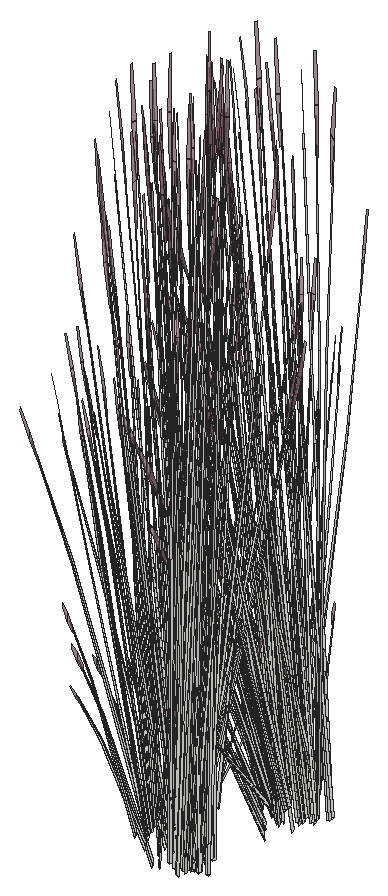
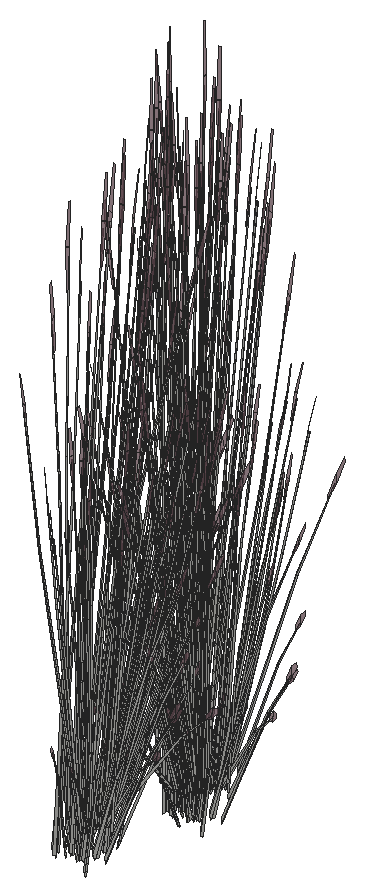
# SketchUp Ruby script. Lengths in inches.
U = 1.inch
M = Sketchup.active_model
def pt(a) = Geom::Point3d.new(a.map { |v| v * U })
def face(e, loops, mat)
  f = e.add_face(loops[0].map { |a| pt(a) })
  loops[1..].each { |l| e.add_face(l.map { |a| pt(a) }).erase! }
  f.material = f.back_material = mat if mat
  f
end
# faces: each face lists its corners as indices into pts; further lists are holes
def faces(e, pts, list, mat = nil) = list.each { |f| face(e, (f[0].is_a?(Array) ? f : [f]).map { |l| l.map { |i| pts[i] } }, mat) }
# xy, xz, yz: faces in a plane at the given z, y or x. An outline is a flat list of corners, or four numbers for a rectangle; further outlines are holes
def ring(l) = l.size == 4 ? [[l[0], l[1]], [l[2], l[1]], [l[2], l[3]], [l[0], l[3]]] : l.each_slice(2).to_a
def flat(e, list, mat, &to3) = list.each { |f| face(e, (f[0].is_a?(Array) ? f : [f]).map { |l| ring(l).map { |u, v| to3.(u, v) } }, mat) }
def xy(e, z, list, mat = nil) = flat(e, list, mat) { |x, y| [x, y, z] }
def xz(e, y, list, mat = nil) = flat(e, list, mat) { |x, z| [x, y, z] }
def yz(e, x, list, mat = nil) = flat(e, list, mat) { |y, z| [x, y, z] }
def lines(e, pts, list) = list.each { |a, b| e.add_line(pt(pts[a]), pt(pts[b])) }
# prism: a flat outline (further loops are holes) pulled along v
def prism(e, loops, v, mat = nil)
  f = face(e, loops, mat); d = Geom::Vector3d.new(v.map { |x| x * U })
  f.pushpull(f.normal.samedirection?(d) ? d.length : -d.length)
end
def box(e, o, s, mat = nil) = prism(e, [[o, [o[0] + s[0], o[1], o[2]], [o[0] + s[0], o[1] + s[1], o[2]], [o[0], o[1] + s[1], o[2]]]], [0, 0, s[2]], mat)
def at(x, y, z, deg = 0) = Geom::Transformation.translation(pt([x, y, z])) * Geom::Transformation.rotation(ORIGIN, Z_AXIS, deg.degrees)
def axes(o, x, y, z) = Geom::Transformation.new([*x, 0, *y, 0, *z, 0, *pt(o).to_a, 1])
def part(name) = M.definitions.add(name)
# library, detail: a bought-in or finely detailed component or shape, given as its bounding box
def library(name, o, s) = part(name).tap { |d| box(d.entities, o, s) }
def detail(e, o, s) = box(e.add_group.entities, o, s)
def put(e, d, t, mat = nil) = e.add_instance(d, t).tap { |i| i.material = mat if mat }
def group(e, t, mat = nil) = e.add_group.tap { |g| g.transformation = t; g.material = mat if mat }.entities
root = M.entities
M.materials.add("LightPink_Translucent").color = [144, 107, 117]
M.materials["LightPink_Translucent"].alpha = 0.75
c1 = part("blade")
p = [[2.15,0.21,22],[0,0.17,0],[0.09,0.45,0],[2.18,0.31,22],[2.29,0.31,22],[0.38,0.45,0],
  [2.48,0.24,33],[2.49,0.24,33],[2.48,0.22,33]]
faces(c1.entities,p,[[0,1,2,3],[4,5,2,3],[6,3,4,7],[8,0,3,6]])
c2 = part("seeds")
p = [[0.3,-0.1,1.38],[-0.01,-0.03,1.59],[-0.01,-0.03,0.03],[0.14,-0.07,-0.07],[0.29,-0.03,3],[0.15,0.01,3.11]]
faces(c2.entities,p,[[0,1,2,3],[1,0,4,5]],"LightPink_Translucent")
c3 = part("blade with seeds")
put(c3.entities,c1,at(0,0,0))
put(c3.entities,c2,axes([2.4,0.25,30.99],[1.5799,-0.05474,1.17369],[-0.12525,1.92788,0.29478],[-0.07173,-0.02425,1.56792]))
put(root,c3,axes([316.24,325.63,275.875],[0.20841,-0.0122,1.71376],[-0.13825,0.52864,0.13857],[-0.297,-0.0327,0.73262]))
put(root,c3,axes([316.33,326.56,275.875],[0.17434,-0.11391,1.71376],[0.14677,0.52637,0.13857],[-0.27369,0.11897,0.73262]))
put(root,c3,axes([315.78,327.46,274.59],[0.17462,0.04421,1.43002],[0.11254,0.45156,-0.30754],[-0.23719,0.08453,0.61141]))
put(root,c3,axes([317.33,326.01,275.34],[0.14282,-0.0779,1.77064],[0.04925,0.54394,0.13857],[-0.30935,0.07218,0.63284]))
put(root,c3,axes([315.79,326.375,276.72],[-0.08205,0.06992,1.74944],[0.00698,0.51086,-0.27667],[-0.18807,0.06644,0.14031]))
put(root,c3,axes([316.06,326.08,276.53],[-0.41757,-0.15024,-0.35414],[0.12179,-0.4383,0.4572],[-0.16812,0.04019,0.87481]))
put(root,c3,axes([314.88,326.89,276.71],[0.06412,0.01444,1.77383],[0.19837,0.47583,-0.16761],[-0.13126,0.12489,0.31391]))
put(root,c3,axes([316.34,326.31,276.68],[-0.13612,0.48987,-0.51099],[-0.46669,-0.16791,-0.3958],[-0.1879,0.04492,0.97773]))
put(root,c3,axes([316.7,325.25,276.68],[-0.36484,0.35674,-0.51099],[-0.31952,-0.37685,-0.3958],[-0.18537,-0.05428,0.97773]))
put(root,c3,axes([316.11,326.28,273.49],[0.01274,0.08487,1.76342],[-0.25688,0.44323,-0.26939],[-0.18246,-0.02234,0.30037]))
put(root,c3,axes([316.18,324.25,276.71],[0.03725,0.05374,1.77383],[-0.17957,0.48312,-0.16761],[-0.18186,0.0035,0.31391]))
put(root,c3,axes([315.42,328.4,274.77],[0.2094,-0.24408,1.1486],[0.08263,0.38639,0.84392],[-0.15132,0.06919,0.25299]))
put(root,c3,axes([316.15,326.03,276.73],[0.14195,-0.49104,0.48003],[0.46669,0.16791,0.3958],[-0.18353,0.02951,0.9933]))
put(root,c3,axes([316.32,325.89,277.03],[0.25281,0.48765,-0.1216],[-0.44869,0.23964,-0.67495],[-0.18908,0.06434,1.02557]))
put(root,c3,axes([316.89,324.875,277.03],[-0.0269,0.54769,-0.1216],[-0.50939,-0.01497,-0.67495],[-0.19618,-0.03804,1.02557]))
put(root,c3,axes([316.12,325.9,276.73],[-0.18454,-0.3672,0.0643],[0.33652,-0.17973,0.50621],[-0.14834,0.03546,0.77189]))
put(root,c3,axes([316.96,326.91,275.875],[0.1255,-0.16547,1.71376],[0.31687,0.44665,0.13857],[-0.21734,0.2034,0.73262]))
put(root,c3,axes([316.21,327.35,276.53],[-0.43736,0.07697,-0.35414],[-0.11549,-0.43998,0.4572],[-0.12533,0.11818,0.87481]))
put(root,c3,axes([315.97,328.65,273.49],[0.0674,0.0538,1.76342],[0.11428,0.49852,-0.26939],[-0.14937,0.10631,0.30037]))
put(root,c3,axes([315.875,325.72,274.77],[0.32078,-0.03854,1.1486],[-0.20348,0.33954,0.84392],[-0.15852,-0.05093,0.25299]))
put(root,c3,axes([316.27,327.25,276.73],[-0.12461,-0.49565,0.48003],[0.48882,-0.08602,0.3958],[-0.14406,0.11657,0.9933]))
put(root,c3,axes([316.17,327.16,276.73],[-0.34493,-0.22649,0.0643],[0.20082,-0.32253,0.50621],[-0.11059,0.10427,0.77189]))
put(root,c3,axes([316.87,327.32,275.875],[0.09355,-0.18511,1.71376],[0.39247,0.38307,0.13857],[-0.17705,0.23875,0.73262]))
put(root,c3,axes([316.5,326.03,277.05],[0.41757,0.15024,0.35414],[-0.12179,0.4383,-0.4572],[-0.16812,0.04019,0.87481]))
put(root,c3,axes([319.15,335.58,275.875],[0.20841,-0.0122,1.71376],[-0.13825,0.52864,0.13857],[-0.297,-0.0327,0.73262]))
put(root,c3,axes([316.57,327.4,276.68],[0.12908,0.49174,-0.51099],[-0.48882,0.08602,-0.3958],[-0.14008,0.13208,0.97773]))
put(root,c3,axes([315.81,328.28,276.72],[-0.01249,0.10657,1.74944],[0.35444,0.37075,-0.27667],[-0.09279,0.17532,0.14031]))
put(root,c3,axes([317.79,327.05,274.06],[-0.52267,-0.08829,-0.62353],[0.11029,-0.54463,-0.16365],[-0.15598,-0.06599,1.37633]))
put(root,c3,axes([316.97,325.09,277.05],[0.28589,0.33718,0.35414],[-0.32644,0.31919,-0.4572],[-0.16586,-0.04856,0.87481]))
put(root,c3,axes([317.1,328.08,274.02],[-0.47024,-0.26927,-0.49651],[0.28107,-0.48284,0],[-0.1071,-0.06133,1.57504]))
put(root,c3,axes([319.24,336.51,275.875],[0.17434,-0.11391,1.71376],[0.14677,0.52637,0.13857],[-0.27369,0.11897,0.73262]))
put(root,c3,axes([316.34,327.05,277.03],[0.46478,0.29695,-0.1216],[-0.26776,0.43004,-0.67495],[-0.13131,0.14949,1.02557]))
put(root,c3,axes([317.39,328.4,274.375],[-0.31414,0.53965,0],[-0.52557,-0.30095,-0.51607],[-0.1197,-0.06854,1.63711]))
put(root,c3,axes([318.7,337.4,274.59],[0.17462,0.04421,1.43002],[0.11254,0.45156,-0.30754],[-0.23719,0.08453,0.61141]))
put(root,c3,axes([320.24,335.96,275.34],[0.14282,-0.0779,1.77064],[0.04925,0.54394,0.13857],[-0.30935,0.07218,0.63284]))
put(root,c3,axes([315.57,328.34,277.65],[0.44338,0.14375,-0.06488],[-0.13639,0.44245,-0.29416],[-0.07252,0.06718,0.97024]))
put(root,c3,axes([316.57,327.09,277.05],[0.43736,-0.07697,0.35414],[0.11549,0.43998,-0.4572],[-0.12533,0.11818,0.87481]))
put(root,c3,axes([316.82,329.18,274.59],[0.15856,-0.08496,1.43002],[0.39147,0.25616,-0.30754],[-0.11652,0.22165,0.61141]))
put(root,c3,axes([318.7,336.32,276.72],[-0.08205,0.06992,1.74944],[0.00698,0.51086,-0.27667],[-0.18807,0.06644,0.14031]))
put(root,c3,axes([319.77,335.08,276.98],[-0.50227,-0.01297,-0.71045],[0.03373,-0.54602,0.08574],[-0.21278,-0.05762,1.00501]))
put(root,c3,axes([319.37,335.22,274.59],[0.0981,0.14994,1.43002],[-0.22605,0.40756,-0.30754],[-0.23211,-0.09741,0.61141]))
put(root,c3,axes([318.38,327.125,274.67],[-0.5073,0.35754,-0.29095],[-0.33735,-0.5052,-0.50002],[-0.12516,-0.05131,1.59708]))
put(root,c3,axes([318.97,336.03,276.53],[-0.41757,-0.15024,-0.35414],[0.12179,-0.4383,0.4572],[-0.16812,0.04019,0.87481]))
put(root,c3,axes([316.98,328.25,276.73],[-0.35779,-0.36745,0.48003],[0.37996,-0.3169,0.3958],[-0.066,0.17239,0.9933]))
put(root,c3,axes([319.55,334.73,275.875],[0.18664,0.09279,1.71376],[-0.38624,0.38925,0.13857],[-0.24072,-0.1756,0.73262]))
put(root,c3,axes([317.23,327.875,274.03],[-0.11803,-0.46926,-0.30978],[0.46876,-0.13325,0.30978],[-0.0945,-0.05411,1.38974]))
put(root,c3,axes([316.85,328.22,276.73],[-0.4129,-0.02509,0.0643],[0.01132,-0.37891,0.50621],[-0.04321,0.14514,0.77189]))
put(root,c3,axes([316.98,328.37,276.53],[-0.33997,0.28354,-0.35414],[-0.32182,-0.32376,0.4572],[-0.04897,0.1645,0.87481]))
put(root,c3,axes([317.79,336.84,276.71],[0.06412,0.01444,1.77383],[0.19837,0.47583,-0.16761],[-0.13126,0.12489,0.31391]))
put(root,c3,axes([319.25,336.25,276.68],[-0.13612,0.48987,-0.51099],[-0.46669,-0.16791,-0.3958],[-0.1879,0.04492,0.97773]))
put(root,c3,axes([319.61,335.19,276.68],[-0.36484,0.35674,-0.51099],[-0.31952,-0.37685,-0.3958],[-0.18537,-0.05428,0.97773]))
put(root,c3,axes([319.02,336.22,273.49],[0.01274,0.08487,1.76342],[-0.25688,0.44323,-0.26939],[-0.18246,-0.02234,0.30037]))
put(root,c3,axes([318.72,327.52,274.06],[-0.33843,0.40479,-0.62353],[-0.42041,-0.36705,-0.16365],[-0.13561,0.10098,1.37633]))
put(root,c3,axes([315.77,329.375,276.71],[0.057,-0.03251,1.77383],[0.47114,0.21627,-0.16761],[-0.01107,0.18007,0.31391]))
put(root,c3,axes([319.09,334.19,276.71],[0.03725,0.05374,1.77383],[-0.17957,0.48312,-0.16761],[-0.18186,0.0035,0.31391]))
put(root,c3,axes([318.33,338.35,274.77],[0.2094,-0.24408,1.1486],[0.08263,0.38639,0.84392],[-0.15132,0.06919,0.25299]))
put(root,c3,axes([318.95,327.29,274.46],[-0.49063,-0.43346,-0.25192],[0.41285,-0.48673,0.5513],[-0.13212,0.05071,1.68216]))
put(root,c3,axes([318.06,326.87,274.21],[-0.30184,-0.45202,-0.44739],[0.45719,-0.31831,0.21531],[-0.09768,-0.05593,1.43643]))
put(root,c3,axes([319.51,333.87,276.72],[-0.10811,-0.0038,1.74944],[-0.34418,0.38014,-0.27667],[-0.18364,-0.07767,0.14031]))
put(root,c3,axes([317.21,328.07,277.34],[-0.01307,0.49815,-0.7886],[-0.55054,-0.03346,0.09517],[-0.0581,0.21104,1.11556]))
put(root,c3,axes([319.06,335.98,276.73],[0.14195,-0.49104,0.48003],[0.46669,0.16791,0.3958],[-0.18353,0.02951,0.9933]))
put(root,c3,axes([319.23,335.83,277.03],[0.25281,0.48765,-0.1216],[-0.44869,0.23964,-0.67495],[-0.18908,0.06434,1.02557]))
put(root,c3,axes([317.2,329.47,274.77],[-0.013,-0.32022,1.1486],[0.32493,0.22839,0.84392],[-0.0639,0.15263,0.25299]))
put(root,c3,axes([319.8,334.82,277.03],[-0.0269,0.54769,-0.1216],[-0.50939,-0.01497,-0.67495],[-0.19618,-0.03804,1.02557]))
put(root,c3,axes([319.47,334.86,276.53],[-0.28589,-0.33718,-0.35414],[0.32644,-0.31919,0.4572],[-0.16586,-0.04856,0.87481]))
put(root,c3,axes([318.7,327.2,274.21],[-0.54562,0.03324,-0.44739],[-0.04934,-0.55185,0.21531],[-0.09768,0.05593,1.43643]))
put(root,c3,axes([319.03,335.84,276.73],[-0.18454,-0.3672,0.0643],[0.33652,-0.17973,0.50621],[-0.14834,0.03546,0.77189]))
put(root,c3,axes([319.875,336.86,275.875],[0.1255,-0.16547,1.71376],[0.31687,0.44665,0.13857],[-0.21734,0.2034,0.73262]))
put(root,c3,axes([319.12,337.29,276.53],[-0.43736,0.07697,-0.35414],[-0.11549,-0.43998,0.4572],[-0.12533,0.11818,0.87481]))
put(root,c3,axes([318.88,338.6,273.49],[0.0674,0.0538,1.76342],[0.11428,0.49852,-0.26939],[-0.14937,0.10631,0.30037]))
put(root,c3,axes([318.79,335.67,274.77],[0.32078,-0.03854,1.1486],[-0.20348,0.33954,0.84392],[-0.15852,-0.05093,0.25299]))
put(root,c3,axes([317.66,328.12,274.48],[0.47024,0.26927,0.49651],[-0.28107,0.48284,0],[-0.1071,-0.06133,1.57504]))
put(root,c3,axes([317.02,328.77,275.36],[0.01104,-0.27801,1.54345],[0.49652,0.14685,0.21329],[-0.04302,0.2963,0.72882]))
put(root,c3,axes([318.1,327.13,274.4375],[0.13317,-0.63814,-0.23429],[0.63143,0.11124,0.51271],[-0.11033,-0.08813,1.5644]))
put(root,c3,axes([319.18,337.2,276.73],[-0.12461,-0.49565,0.48003],[0.48882,-0.08602,0.3958],[-0.14406,0.11657,0.9933]))
put(root,c3,axes([318.33,327.28,274.62],[-0.09693,0.48062,0.1448],[-0.47357,-0.08343,-0.41347],[-0.08619,-0.04935,1.26744]))
put(root,c3,axes([319.43,334.73,277.09],[0.41494,-0.39744,0.53763],[0.35786,0.42207,0.4433],[-0.19468,-0.07331,1.11249]))
put(root,c3,axes([319.28,328.62,274.02],[-0.47024,0.26927,-0.49651],[-0.28107,-0.48284,0],[-0.1071,0.06133,1.57504]))
put(root,c3,axes([316.73,326.4375,274.48],[0,0.53854,0.49651],[-0.56215,0,0],[0,-0.12266,1.57504]))
put(root,c3,axes([319.08,337.1,276.73],[-0.34493,-0.22649,0.0643],[0.20082,-0.32253,0.50621],[-0.11059,0.10427,0.77189]))
put(root,c3,axes([319.31,328.48,274.19],[-0.31023,-0.54153,-0.05142],[0.52557,-0.30095,0.51607],[-0.12951,0.05156,1.6363]))
put(root,c3,axes([317.32,328.23,277],[0.35968,0.36185,-0.5672],[-0.37996,0.3169,-0.43934],[-0.05473,0.18385,1.08528]))
put(root,c3,axes([319.78,337.27,275.875],[0.09355,-0.18511,1.71376],[0.39247,0.38307,0.13857],[-0.17705,0.23875,0.73262]))
put(root,c3,axes([319.17,328.41,274.03],[-0.46876,-0.13325,-0.30978],[0.11803,-0.46926,0.30978],[-0.0945,0.05411,1.38974]))
put(root,c3,axes([317.16,327.96,277.05],[0.33997,-0.28354,0.35414],[0.32182,0.32376,-0.4572],[-0.04897,0.1645,0.87481]))
put(root,c3,axes([319.44,326.4,274.84],[-0.01373,-0.50706,1.41272],[0.62119,0.13144,0.59816],[-0.14692,0.27746,1.3335]))
put(root,c3,axes([319.41,335.98,277.05],[0.41757,0.15024,0.35414],[-0.12179,0.4383,-0.4572],[-0.16812,0.04019,0.87481]))
put(root,c3,axes([319.48,337.34,276.68],[0.12908,0.49174,-0.51099],[-0.48882,0.08602,-0.3958],[-0.14008,0.13208,0.97773]))
put(root,c3,axes([316.94,328.04,277.4],[0.55221,0.02668,-0.13498],[-0.01509,0.50521,-0.74919],[-0.03836,0.19458,1.13838]))
put(root,c3,axes([316.93,328.77,274.82],[0.45645,-0.09537,0.06507],[0.10494,0.38421,-0.86304],[-0.02894,0.19449,0.7736]))
put(root,c3,axes([319.62,334.73,276.73],[0.0253,-0.40952,0.0643],[0.38204,0.01123,0.50621],[-0.14634,-0.04285,0.77189]))
put(root,c3,axes([318.72,338.23,276.72],[-0.01249,0.10657,1.74944],[0.35444,0.37075,-0.27667],[-0.09279,0.17532,0.14031]))
put(root,c3,axes([319.09,327.05,274.67],[0.05855,0.61451,-0.29095],[-0.60981,0.03716,-0.50002],[-0.10738,0.08185,1.59708]))
put(root,c3,axes([320.7,336.99,274.06],[-0.52267,-0.08829,-0.62353],[0.11029,-0.54463,-0.16365],[-0.15598,-0.06599,1.37633]))
put(root,c3,axes([320.79,334.02,277.43],[-0.33533,0.51628,-0.13619],[-0.48563,-0.29744,-0.75594],[-0.16881,-0.14586,1.14864]))
put(root,c3,axes([319.88,335.04,277.05],[0.28589,0.33718,0.35414],[-0.32644,0.31919,-0.4572],[-0.16586,-0.04856,0.87481]))
put(root,c3,axes([317.73,327.71,275.875],[-0.0123,-0.2067,1.71376],[0.53301,0.13712,0.13857],[-0.03297,0.29456,0.73262]))
put(root,c3,axes([320.65,334.44,276.98],[-0.42844,-0.2603,-0.71045],[0.30448,-0.45614,0.08574],[-0.15523,-0.15542,1.00501]))
put(root,c3,axes([320.45,334.45,276.68],[-0.4958,0.12802,-0.51099],[-0.08673,-0.48481,-0.3958],[-0.13317,-0.13893,0.97773]))
put(root,c3,axes([318.18,326.82,274.36],[0.63506,0.11347,0.45755],[-0.12924,0.64083,0.17955],[-0.09281,-0.06188,1.58856]))
put(root,c3,axes([320.01,338.02,274.02],[-0.47024,-0.26927,-0.49651],[0.28107,-0.48284,0],[-0.1071,-0.06133,1.57504]))
put(root,c3,axes([319.81,334.01,273.49],[-0.04867,0.07094,1.76342],[-0.49185,0.15296,-0.26939],[-0.11882,-0.13915,0.30037]))
put(root,c3,axes([319.25,336.99,277.03],[0.46478,0.29695,-0.1216],[-0.26776,0.43004,-0.67495],[-0.13131,0.14949,1.02557]))
put(root,c3,axes([318.01,326.71,274.72],[-0.24378,0.48527,0.44739],[-0.50654,-0.23354,-0.21531],[0,-0.11186,1.43643]))
put(root,c3,axes([320.3,338.35,274.375],[-0.31414,0.53965,0],[-0.52557,-0.30095,-0.51607],[-0.1197,-0.06854,1.63711]))
put(root,c3,axes([317.84,327.85,274.47],[0.53992,-0.14294,0.17642],[0.13332,0.53195,0.35086],[-0.04815,-0.07751,1.60407]))
put(root,c3,axes([318.48,338.28,277.65],[0.44338,0.14375,-0.06488],[-0.13639,0.44245,-0.29416],[-0.07252,0.06718,0.97024]))
put(root,c3,axes([318.53,327.93,274.2],[-0.50654,-0.24178,0],[0.24378,-0.50239,0],[0,0,1.62707]))
put(root,c3,axes([319.48,337.03,277.05],[0.43736,-0.07697,0.35414],[0.11549,0.43998,-0.4572],[-0.12533,0.11818,0.87481]))
put(root,c3,axes([319.7,328.54,274.375],[0.31414,0.53965,0],[-0.52557,0.30095,-0.51607],[-0.1197,0.06854,1.63711]))
put(root,c3,axes([318.1,328.77,277.0625],[-0.4951,-0.14079,0.53283],[0.1693,-0.46287,0.43934],[0.02975,0.18203,1.10256]))
put(root,c3,axes([319.5,334.29,274.13],[-0.14494,0.43975,-0.03893],[-0.4461,-0.13527,-0.17649],[-0.06773,-0.07192,0.58215]))
put(root,c3,axes([317.97,328.8,276.73],[-0.37023,0.18303,0.0643],[-0.18122,-0.33376,0.50621],[0.03575,0.14712,0.77189]))
put(root,c3,axes([320.66,332.79,276.71],[-0.00937,0.06455,1.77383],[-0.46231,0.23427,-0.16761],[-0.13604,-0.11975,0.31391]))
put(root,c3,axes([319.44,327.875,274.47],[0.14515,-0.53522,0.17642],[0.53115,0.15146,0.35086],[-0.09175,0.00261,1.60407]))
put(root,c3,axes([319.2,327.17,274.62],[0.37121,0.32357,0.1448],[-0.30963,0.36505,-0.41347],[-0.08619,0.04935,1.26744]))
put(root,c3,axes([320.17,333.73,274.59],[-0.03043,0.17617,1.43002],[-0.4448,0.14748,-0.30754],[-0.10397,-0.22771,0.61141]))
put(root,c3,axes([319.07,326.77,274.3],[-0.46736,-0.46353,-0.06131],[0.46764,-0.46381,0],[-0.01632,-0.01619,1.75571]))
put(root,c3,axes([320.3125,334.1875,275.875],[0.11485,0.17291,1.71376],[-0.53072,0.14557,0.13857],[-0.11995,-0.27145,0.73262]))
put(root,c3,axes([319.1875,326.93,274.72],[0.54562,-0.03324,0.44739],[0.04934,0.55185,-0.21531],[-0.09768,0.05593,1.43643]))
put(root,c3,axes([321.29,337.07,274.67],[-0.5073,0.35754,-0.29095],[-0.33735,-0.5052,-0.50002],[-0.12516,-0.05131,1.59708]))
put(root,c3,axes([319.89,338.2,276.73],[-0.35779,-0.36745,0.48003],[0.37996,-0.3169,0.3958],[-0.066,0.17239,0.9933]))
put(root,c3,axes([319.32,328.2,274.33],[0.62903,0.17504,0.30756],[-0.15737,0.62568,-0.36492],[-0.10411,0.07831,1.64885]))
put(root,c3,axes([320.5,334.1,276.53],[-0.0776,-0.43378,-0.35414],[0.44361,-0.11454,0.4572],[-0.11915,-0.12431,0.87481]))
put(root,c3,axes([319.26,336.29,274.375],[-0.62828,0,0],[0,-0.6019,-0.51607],[0,-0.13709,1.63711]))
put(root,c3,axes([320.15,337.82,274.03],[-0.11803,-0.46926,-0.30978],[0.46876,-0.13325,0.30978],[-0.0945,-0.05411,1.38974]))
put(root,c3,axes([319.76,338.17,276.73],[-0.4129,-0.02509,0.0643],[0.01132,-0.37891,0.50621],[-0.04321,0.14514,0.77189]))
put(root,c3,axes([319.59,328.16,274.48],[0.47024,-0.26927,0.49651],[0.28107,0.48284,0],[-0.1071,0.06133,1.57504]))
put(root,c3,axes([319.89,338.3125,276.53],[-0.33997,0.28354,-0.35414],[-0.32182,-0.32376,0.4572],[-0.04897,0.1645,0.87481]))
put(root,c3,axes([318.12,326.23,274.36],[0.21845,0.6022,0.45755],[-0.62418,0.20941,0.17955],[0.00763,-0.11065,1.58856]))
put(root,c3,axes([318.65,327.72,274.2],[-0.16394,-0.4643,0],[0.46814,-0.1626,0],[0,0,1.54371]))
put(root,c3,axes([318.05,328.7,273.49],[0.08132,-0.0293,1.76342],[0.48914,0.1613,-0.26939],[0.0143,0.18179,0.30037]))
put(root,c3,axes([318.16,328.87,276.53],[-0.15148,0.41415,-0.35414],[-0.44193,-0.12079,0.4572],[0.04052,0.16674,0.87481]))
put(root,c3,axes([321.63,337.46,274.06],[-0.33843,0.40479,-0.62353],[-0.42041,-0.36705,-0.16365],[-0.13561,0.10098,1.37633]))
put(root,c3,axes([320.76,334.45,277.05],[0.0776,0.43378,0.35414],[-0.44361,0.11454,-0.4572],[-0.11915,-0.12431,0.87481]))
put(root,c3,axes([319.75,336.13,274.33],[-0.46736,0.45277,0.30756],[-0.46764,-0.44801,-0.36492],[-0.01632,-0.12858,1.64885]))
put(root,c3,axes([321.67,337.39,275.33],[0.4342,0.21716,1.51261],[-0.42537,0.46784,0.59816],[-0.19053,-0.27728,1.26806]))
put(root,c3,axes([320.02,333.45,274.77],[0.2621,0.18744,1.1486],[-0.38171,0.11267,0.84392],[-0.08167,-0.14405,0.25299]))
put(root,c3,axes([321.86,337.24,274.46],[-0.49063,-0.43346,-0.25192],[0.41285,-0.48673,0.5513],[-0.13212,0.05071,1.68216]))
put(root,c3,axes([319.31,326.81,274.21],[-0.24378,0.48527,-0.44739],[-0.50654,-0.23354,0.21531],[0,0.11186,1.43643]))
put(root,c3,axes([320.97,336.82,274.21],[-0.30184,-0.45202,-0.44739],[0.45719,-0.31831,0.21531],[-0.09768,-0.05593,1.43643]))
put(root,c3,axes([317.85,329.6,276.72],[0.06369,0.08672,1.74944],[0.51399,0.03407,-0.27667],[0.05169,0.19126,0.14031]))
put(root,c3,axes([320.27,326.51,274.47],[-0.39477,-0.39228,0.17642],[0.39783,-0.38049,0.35086],[-0.0436,0.08011,1.60407]))
put(root,c3,axes([320.11,339.41,274.77],[-0.013,-0.32022,1.1486],[0.32493,0.22839,0.84392],[-0.0639,0.15263,0.25299]))
put(root,c3,axes([320.5625,333.9375,277.09],[0.55971,-0.13842,0.53763],[0.09714,0.54299,0.4433],[-0.13164,-0.16003,1.11249]))
put(root,c3,axes([318.91,326.28,274.21],[0,-0.62313,0],[0.62828,0,0],[0,0,1.79456]))
put(root,c3,axes([321.61,337.14,274.21],[-0.54562,0.03324,-0.44739],[-0.04934,-0.55185,0.21531],[-0.09768,0.05593,1.43643]))
put(root,c3,axes([318.32,326.4,274.43],[0.56613,0.26102,0.24065],[-0.27246,0.54236,0.50002],[0,-0.12502,1.60543]))
put(root,c3,axes([319.22,326.53,274.29],[0,0.62282,-0.05637],[-0.62828,0,0],[0,0.01957,1.79368]))
put(root,c3,axes([318.14,326.03,274.72],[-0.54562,0.03324,0.44739],[-0.04934,-0.55185,-0.21531],[0.09768,-0.05593,1.43643]))
put(root,c3,axes([318.11,328.43,277.05],[0.15148,-0.41415,0.35414],[0.44193,0.12079,-0.4572],[0.04052,0.16674,0.87481]))
put(root,c3,axes([320.69,334.06,276.73],[0.22836,-0.34211,0.0643],[0.3252,0.19918,0.50621],[-0.10513,-0.10968,0.77189]))
put(root,c3,axes([317.89,325.09,274.47],[-0.14515,0.53522,0.17642],[-0.53115,-0.15146,0.35086],[0.09175,-0.00261,1.60407]))
put(root,c3,axes([318.92,327.74,274.29],[0.21845,0.61869,-0.06012],[-0.62418,0.21679,0],[0.00763,0.02161,1.72173]))
put(root,c3,axes([320.57,338.07,274.48],[0.47024,0.26927,0.49651],[-0.28107,0.48284,0],[-0.1071,-0.06133,1.57504]))
put(root,c3,axes([321.02,337.08,274.4375],[0.13317,-0.63814,-0.23429],[0.63143,0.11124,0.51271],[-0.11033,-0.08813,1.5644]))
put(root,c3,axes([321.24,337.23,274.62],[-0.09693,0.48062,0.1448],[-0.47357,-0.08343,-0.41347],[-0.08619,-0.04935,1.26744]))
put(root,c3,axes([318.2,328.49,276.98],[0.23981,0.43789,-0.71045],[-0.49365,0.24404,0.08574],[0.05608,0.21158,1.00501]))
put(root,c3,axes([320.73,326.93,274.2],[-0.62797,-0.00431,-0.04976],[0,-0.6019,0.49943],[-0.01973,0.13702,1.58352]))
put(root,c3,axes([321.19,333.04,276.72],[-0.07685,-0.07551,1.74944],[-0.51287,0.04787,-0.27667],[-0.08185,-0.1806,0.14031]))
put(root,c3,axes([322.1875,338.57,274.02],[-0.47024,0.26927,-0.49651],[-0.28107,-0.48284,0],[-0.1071,0.06133,1.57504]))
put(root,c3,axes([319.4,335.88,274.02],[0,-0.53854,-0.49651],[0.56215,0,0],[0,-0.12266,1.57504]))
put(root,c3,axes([319.64,336.38,274.48],[0,0.53854,0.49651],[-0.56215,0,0],[0,-0.12266,1.57504]))
put(root,c3,axes([322.22,338.42,274.19],[-0.31023,-0.54153,-0.05142],[0.52557,-0.30095,0.51607],[-0.12951,0.05156,1.6363]))
put(root,c3,axes([319.49,325.12,274.47],[-0.53992,0.14294,0.17642],[-0.13332,-0.53195,0.35086],[0.04815,0.07751,1.60407]))
put(root,c3,axes([318.7,329.91,277.65],[0.34721,-0.30895,-0.06488],[0.31814,0.33837,-0.29416],[0.0224,0.09588,0.97024]))
put(root,c3,axes([322.08,338.35,274.03],[-0.46876,-0.13325,-0.30978],[0.11803,-0.46926,0.30978],[-0.0945,0.05411,1.38974]))
put(root,c3,axes([318.61,325.89,274.36],[-0.4166,0.48873,0.45755],[-0.49494,-0.43142,0.17955],[0.10044,-0.04877,1.58856]))
put(root,c3,axes([320.07,337.91,277.05],[0.33997,-0.28354,0.35414],[0.32182,0.32376,-0.4572],[-0.04897,0.1645,0.87481]))
put(root,c3,axes([319.32,326.66,274.21],[0.35073,0.34786,0],[-0.35073,0.34786,0],[0,0,1.69266]))
put(root,c3,axes([319.32,326.26,274.72],[0.24378,-0.48527,0.44739],[0.50654,0.23354,-0.21531],[0,0.11186,1.43643]))
put(root,c3,axes([319.11,327.94,274.2],[0.50654,0.24178,0],[-0.24378,0.50239,0],[0,0,1.74954]))
put(root,c3,axes([320.87,336.51,274.67],[-0.56585,-0.25696,-0.29095],[0.27246,-0.54236,-0.50002],[-0.01778,-0.13316,1.59708]))
put(root,c3,axes([322.35,336.35,274.84],[-0.01373,-0.50706,1.41272],[0.62119,0.13144,0.59816],[-0.14692,0.27746,1.3335]))
put(root,c3,axes([318.38,328.58,276.68],[0.49392,0.135,-0.51099],[-0.1693,0.46287,-0.3958],[0.04529,0.18636,0.97773]))
put(root,c3,axes([317.96,328.6,277.03],[0.49168,-0.25073,-0.1216],[0.24162,0.44501,-0.67495],[0.06487,0.18753,1.02557]))
put(root,c3,axes([319.15,326.14,274.38],[-0.63506,-0.11347,0.49198],[0.12924,-0.64083,0.19306],[0.09281,0.06188,1.70813]))
put(root,c3,axes([319.85,337.99,277.4],[0.55221,0.02668,-0.13498],[-0.01509,0.50521,-0.74919],[-0.03836,0.19458,1.13838]))
put(root,c3,axes([322,336.99,274.67],[0.05855,0.61451,-0.29095],[-0.60981,0.03716,-0.50002],[-0.10738,0.08185,1.59708]))
put(root,c3,axes([320.6,327.01,274.03],[-0.35073,0.33601,-0.30978],[-0.35073,-0.33601,0.30978],[0,0.10823,1.38974]))
put(root,c3,axes([320.62,335.96,274.1],[-0.20635,-0.55225,-0.69835],[0.59439,-0.19889,-0.18329],[-0.02281,-0.18701,1.54149]))
put(root,c3,axes([321.97,334.21,277.03],[-0.49168,0.25073,-0.1216],[-0.24162,-0.44501,-0.67495],[-0.06487,-0.18753,1.02557]))
put(root,c3,axes([321.55,334.23,276.68],[-0.49392,-0.135,-0.51099],[0.1693,-0.46287,-0.3958],[-0.04529,-0.18636,0.97773]))
put(root,c3,axes([319.59,326.95,274.09],[0.18424,0.49308,-0.69212],[-0.53071,0.17758,-0.18165],[0.02036,0.16697,1.52773]))
put(root,c3,axes([319.33,326.42,274.21],[0.56215,0,0],[0,0.55754,0],[0,0,1.78407]))
put(root,c3,axes([318.79,325.81,274.72],[-0.30184,-0.45202,0.44739],[0.45719,-0.31831,-0.21531],[0.09768,0.05593,1.43643]))
put(root,c3,axes([319.64,335.9,274.03],[0.35073,-0.33601,-0.30978],[0.35073,0.33601,0.30978],[0,-0.10823,1.38974]))
put(root,c3,axes([319.53,326.37,274.62],[0.46814,-0.15705,0.1448],[0.16394,0.44848,-0.41347],[0,0.0987,1.26744]))
